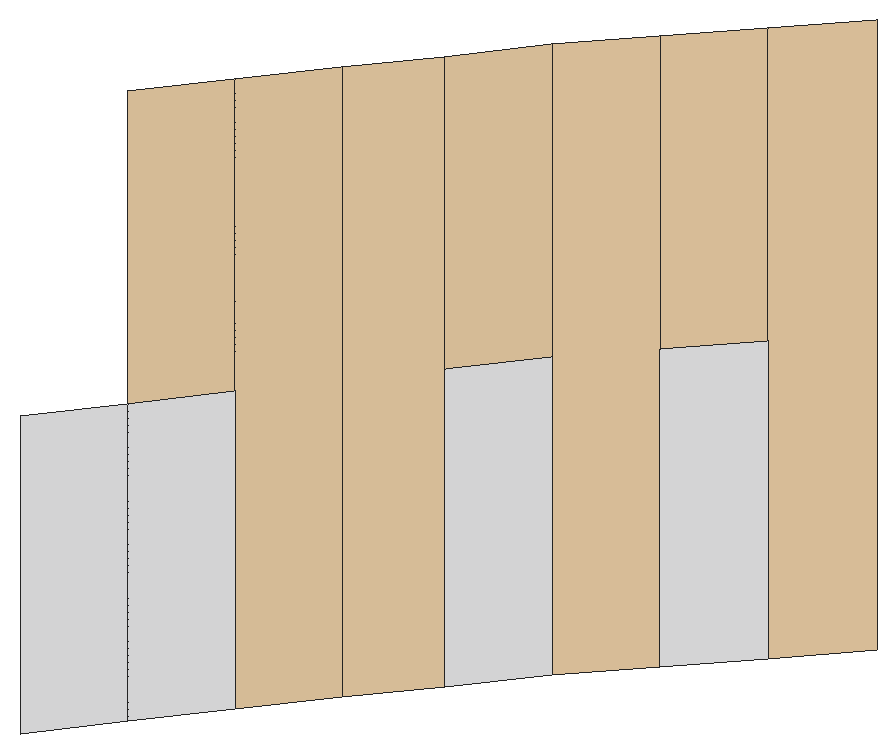
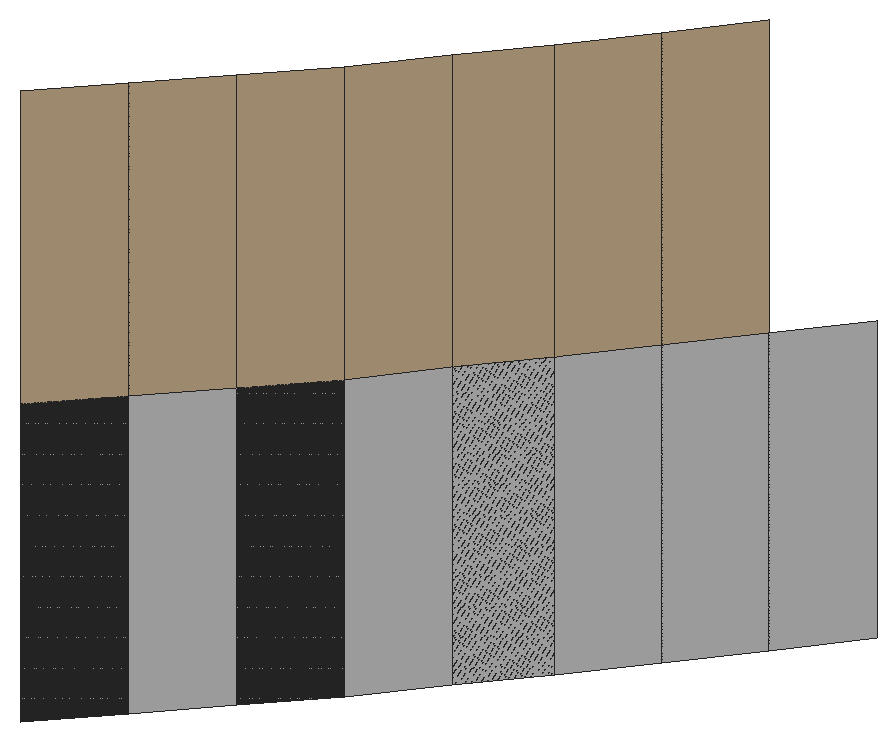
# SketchUp Ruby script. Lengths in inches.
U = 1.inch
M = Sketchup.active_model
def pt(a) = Geom::Point3d.new(a.map { |v| v * U })
def face(e, loops, mat)
  f = e.add_face(loops[0].map { |a| pt(a) })
  loops[1..].each { |l| e.add_face(l.map { |a| pt(a) }).erase! }
  f.material = f.back_material = mat if mat
  f
end
# faces: each face lists its corners as indices into pts; further lists are holes
def faces(e, pts, list, mat = nil) = list.each { |f| face(e, (f[0].is_a?(Array) ? f : [f]).map { |l| l.map { |i| pts[i] } }, mat) }
# xy, xz, yz: faces in a plane at the given z, y or x. An outline is a flat list of corners, or four numbers for a rectangle; further outlines are holes
def ring(l) = l.size == 4 ? [[l[0], l[1]], [l[2], l[1]], [l[2], l[3]], [l[0], l[3]]] : l.each_slice(2).to_a
def flat(e, list, mat, &to3) = list.each { |f| face(e, (f[0].is_a?(Array) ? f : [f]).map { |l| ring(l).map { |u, v| to3.(u, v) } }, mat) }
def xy(e, z, list, mat = nil) = flat(e, list, mat) { |x, y| [x, y, z] }
def xz(e, y, list, mat = nil) = flat(e, list, mat) { |x, z| [x, y, z] }
def yz(e, x, list, mat = nil) = flat(e, list, mat) { |y, z| [x, y, z] }
def lines(e, pts, list) = list.each { |a, b| e.add_line(pt(pts[a]), pt(pts[b])) }
# prism: a flat outline (further loops are holes) pulled along v
def prism(e, loops, v, mat = nil)
  f = face(e, loops, mat); d = Geom::Vector3d.new(v.map { |x| x * U })
  f.pushpull(f.normal.samedirection?(d) ? d.length : -d.length)
end
def box(e, o, s, mat = nil) = prism(e, [[o, [o[0] + s[0], o[1], o[2]], [o[0] + s[0], o[1] + s[1], o[2]], [o[0], o[1] + s[1], o[2]]]], [0, 0, s[2]], mat)
def at(x, y, z, deg = 0) = Geom::Transformation.translation(pt([x, y, z])) * Geom::Transformation.rotation(ORIGIN, Z_AXIS, deg.degrees)
def axes(o, x, y, z) = Geom::Transformation.new([*x, 0, *y, 0, *z, 0, *pt(o).to_a, 1])
def part(name) = M.definitions.add(name)
# library, detail: a bought-in or finely detailed component or shape, given as its bounding box
def library(name, o, s) = part(name).tap { |d| box(d.entities, o, s) }
def detail(e, o, s) = box(e.add_group.entities, o, s)
def put(e, d, t, mat = nil) = e.add_instance(d, t).tap { |i| i.material = mat if mat }
def group(e, t, mat = nil) = e.add_group.tap { |g| g.transformation = t; g.material = mat if mat }.entities
root = M.entities
M.materials.add("False Ceiling Light").color = [254, 223, 179]
M.materials.add("[Quartz Light Grey]").color = [251, 251, 252]
p = [[46.29,212.22,115.32],[46.18,212.08,115.32],[46.18,212.08,115.91],[46.29,212.22,115.91],[46.4,212.36,115.32],[46.4,212.36,115.91],
  [46.29,212.22,115.32],[46.4,212.36,115.32],[46.4,212.36,116.49],[46.29,212.22,116.49],[46.51,212.5,115.32],[46.51,212.5,115.91],
  [46.51,212.5,115.32],[46.51,212.5,116.49],[46.62,212.63,115.32],[46.62,212.63,115.91],[46.62,212.63,115.32],[46.62,212.63,116.49],
  [46.73,212.77,115.32],[46.73,212.77,115.91],[46.73,212.77,115.32],[46.73,212.77,116.49],[46.85,212.9,115.32],[46.85,212.9,115.91],
  [46.85,212.9,115.32],[46.85,212.9,116.49],[46.97,213.03,115.32],[46.97,213.03,115.91],[46.97,213.03,115.32],[46.97,213.03,116.49],
  [47.09,213.16,115.32],[47.09,213.16,115.91],[47.09,213.16,115.32],[47.09,213.16,116.49]]
faces(root,p,[[0,1,2,3],[4,0,3,5],[10,4,5,11],[14,10,11,15],[18,14,15,19],[22,18,19,23],[26,22,23,27],[30,26,27,31]],"[Quartz Light Grey]")
faces(root,p,[[6,7,8,9],[7,12,13,8],[12,16,17,13],[16,20,21,17],[20,24,25,21],[24,28,29,25],[28,32,33,29]],"False Ceiling Light")
